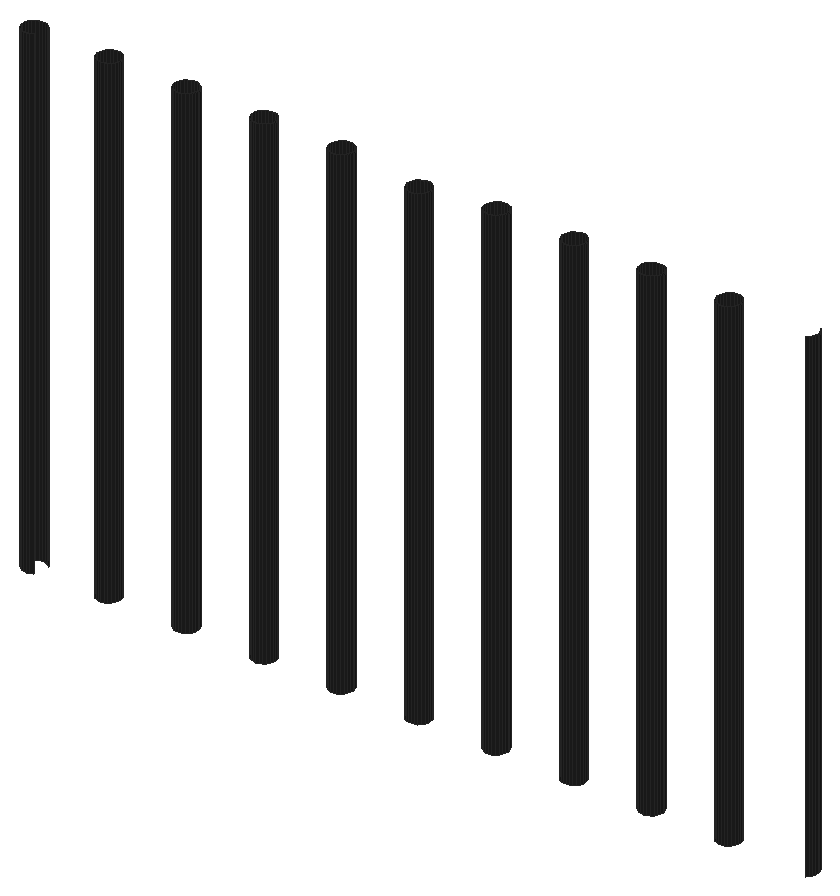
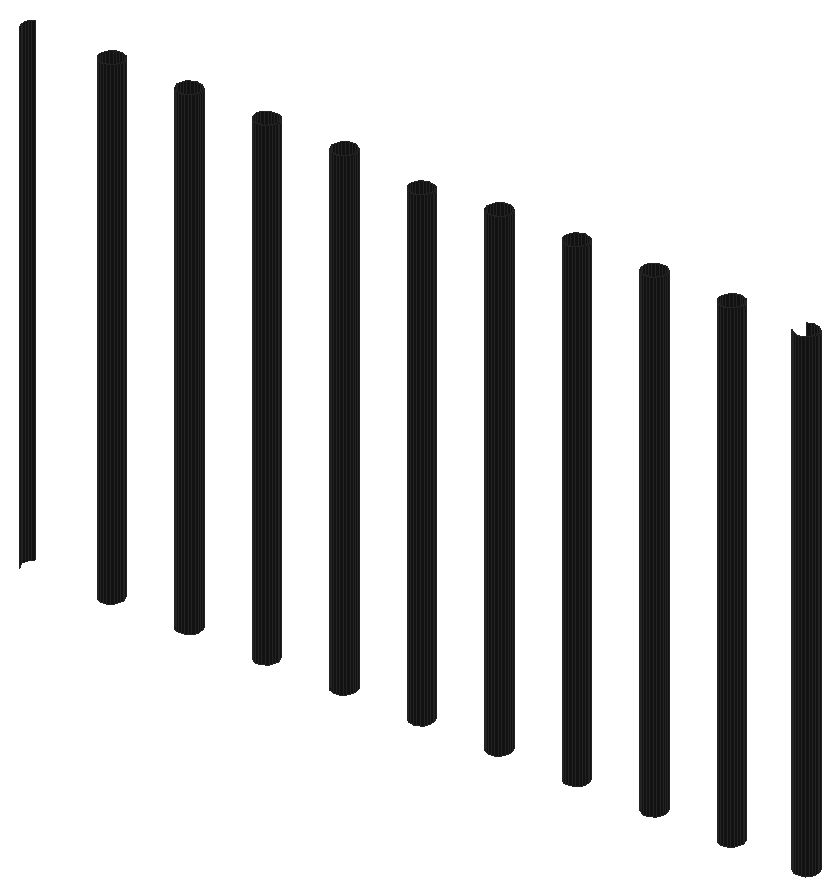
# SketchUp Ruby script. Lengths in inches.
U = 1.inch
M = Sketchup.active_model
def pt(a) = Geom::Point3d.new(a.map { |v| v * U })
def face(e, loops, mat)
  f = e.add_face(loops[0].map { |a| pt(a) })
  loops[1..].each { |l| e.add_face(l.map { |a| pt(a) }).erase! }
  f.material = f.back_material = mat if mat
  f
end
# faces: each face lists its corners as indices into pts; further lists are holes
def faces(e, pts, list, mat = nil) = list.each { |f| face(e, (f[0].is_a?(Array) ? f : [f]).map { |l| l.map { |i| pts[i] } }, mat) }
# xy, xz, yz: faces in a plane at the given z, y or x. An outline is a flat list of corners, or four numbers for a rectangle; further outlines are holes
def ring(l) = l.size == 4 ? [[l[0], l[1]], [l[2], l[1]], [l[2], l[3]], [l[0], l[3]]] : l.each_slice(2).to_a
def flat(e, list, mat, &to3) = list.each { |f| face(e, (f[0].is_a?(Array) ? f : [f]).map { |l| ring(l).map { |u, v| to3.(u, v) } }, mat) }
def xy(e, z, list, mat = nil) = flat(e, list, mat) { |x, y| [x, y, z] }
def xz(e, y, list, mat = nil) = flat(e, list, mat) { |x, z| [x, y, z] }
def yz(e, x, list, mat = nil) = flat(e, list, mat) { |y, z| [x, y, z] }
def lines(e, pts, list) = list.each { |a, b| e.add_line(pt(pts[a]), pt(pts[b])) }
# prism: a flat outline (further loops are holes) pulled along v
def prism(e, loops, v, mat = nil)
  f = face(e, loops, mat); d = Geom::Vector3d.new(v.map { |x| x * U })
  f.pushpull(f.normal.samedirection?(d) ? d.length : -d.length)
end
def box(e, o, s, mat = nil) = prism(e, [[o, [o[0] + s[0], o[1], o[2]], [o[0] + s[0], o[1] + s[1], o[2]], [o[0], o[1] + s[1], o[2]]]], [0, 0, s[2]], mat)
def at(x, y, z, deg = 0) = Geom::Transformation.translation(pt([x, y, z])) * Geom::Transformation.rotation(ORIGIN, Z_AXIS, deg.degrees)
def axes(o, x, y, z) = Geom::Transformation.new([*x, 0, *y, 0, *z, 0, *pt(o).to_a, 1])
def part(name) = M.definitions.add(name)
# library, detail: a bought-in or finely detailed component or shape, given as its bounding box
def library(name, o, s) = part(name).tap { |d| box(d.entities, o, s) }
def detail(e, o, s) = box(e.add_group.entities, o, s)
def put(e, d, t, mat = nil) = e.add_instance(d, t).tap { |i| i.material = mat if mat }
def group(e, t, mat = nil) = e.add_group.tap { |g| g.transformation = t; g.material = mat if mat }.entities
root = M.entities
M.materials.add("[Color M08]").color = [30, 30, 30]
xz(root,194.51,[[121.8,321,122,353.72],[126.86,321,127.06,353.72],[132.11,321,132.31,353.72],[137.36,321,137.56,353.72],[142.61,321,142.81,353.72],
  [147.86,321,148.06,353.1875],[153.11,321,153.31,353.72],[158.36,321,158.56,353.72],[163.61,321,163.81,353.72],[168.86,321,169.06,353.72]],"[Color M08]")
yz(root,126.24,[[195.18,321,195.375,353.72]],"[Color M08]")
yz(root,131.49,[[195.18,321,195.375,353.72]],"[Color M08]")
yz(root,136.74,[[195.18,321,195.375,353.72]],"[Color M08]")
yz(root,141.99,[[195.18,321,195.375,353.72]],"[Color M08]")
yz(root,147.24,[[195.18,321,195.375,353.1875]],"[Color M08]")
yz(root,152.49,[[195.18,321,195.375,353.72]],"[Color M08]")
yz(root,157.74,[[195.18,321,195.375,353.72]],"[Color M08]")
yz(root,162.99,[[195.18,321,195.375,353.72]],"[Color M08]")
yz(root,168.24,[[195.18,321,195.375,353.72]],"[Color M08]")
p = [[121.61,194.57,321],[121.8,194.51,321],[121.8,194.51,353.72],[121.61,194.57,353.72],[122,194.51,321],[122.1875,194.55,321],
  [122.1875,194.55,353.72],[122,194.51,353.72],[126.68,194.57,321],[126.86,194.51,321],[126.86,194.51,353.72],[126.68,194.57,353.72],
  [127.06,194.51,321],[127.25,194.55,321],[127.25,194.55,353.72],[127.06,194.51,353.72],[131.93,194.57,321],[132.11,194.51,321],
  [132.11,194.51,353.72],[131.93,194.57,353.72],[132.31,194.51,321],[132.5,194.55,321],[132.5,194.55,353.72],[132.31,194.51,353.72],
  [137.18,194.57,321],[137.36,194.51,321],[137.36,194.51,353.72],[137.18,194.57,353.72],[137.56,194.51,321],[137.75,194.55,321],
  [137.75,194.55,353.72],[137.56,194.51,353.72],[142.43,194.57,321],[142.61,194.51,321],[142.61,194.51,353.72],[142.43,194.57,353.72],
  [142.81,194.51,321],[143,194.55,321],[143,194.55,353.72],[142.81,194.51,353.72],[147.68,194.57,321],[147.86,194.51,321],
  [147.86,194.51,353.1875],[147.68,194.57,353.1875],[148.06,194.51,321],[148.25,194.55,321],[148.25,194.55,353.1875],[148.06,194.51,353.1875],
  [152.93,194.57,321],[153.11,194.51,321],[153.11,194.51,353.72],[152.93,194.57,353.72],[153.31,194.51,321],[153.5,194.55,321],
  [153.5,194.55,353.72],[153.31,194.51,353.72],[158.18,194.57,321],[158.36,194.51,321],[158.36,194.51,353.72],[158.18,194.57,353.72],
  [158.56,194.51,321],[158.75,194.55,321],[158.75,194.55,353.72],[158.56,194.51,353.72],[163.43,194.57,321],[163.61,194.51,321],
  [163.61,194.51,353.72],[163.43,194.57,353.72],[163.81,194.51,321],[164,194.55,321],[164,194.55,353.72],[163.81,194.51,353.72],
  [168.68,194.57,321],[168.86,194.51,321],[168.86,194.51,353.72],[168.68,194.57,353.72],[169.06,194.51,321],[169.25,194.55,321],
  [169.25,194.55,353.72],[169.06,194.51,353.72],[121.45,194.67,321],[121.45,194.67,353.72],[122.36,194.64,321],[122.36,194.64,353.72],
  [126.51,194.67,321],[126.51,194.67,353.72],[127.42,194.64,321],[127.42,194.64,353.72],[127.5625,194.78,321],[127.5625,194.78,353.72],
  [131.76,194.67,321],[131.76,194.67,353.72],[132.67,194.64,321],[132.67,194.64,353.72],[132.8125,194.78,321],[132.8125,194.78,353.72],
  [137.01,194.67,321],[137.01,194.67,353.72],[137.92,194.64,321],[137.92,194.64,353.72],[138.0625,194.78,321],[138.0625,194.78,353.72],
  [142.26,194.67,321],[142.26,194.67,353.72],[143.17,194.64,321],[143.17,194.64,353.72],[143.3125,194.78,321],[143.3125,194.78,353.72],
  [147.51,194.67,321],[147.51,194.67,353.1875],[148.42,194.64,321],[148.42,194.64,353.1875],[148.5625,194.78,321],[148.5625,194.78,353.1875],
  [152.76,194.67,321],[152.76,194.67,353.72],[153.67,194.64,321],[153.67,194.64,353.72],[153.8125,194.78,321],[153.8125,194.78,353.72],
  [158.01,194.67,321],[158.01,194.67,353.72],[158.92,194.64,321],[158.92,194.64,353.72],[159.0625,194.78,321],[159.0625,194.78,353.72],
  [163.26,194.67,321],[163.26,194.67,353.72],[164.17,194.64,321],[164.17,194.64,353.72],[164.3125,194.78,321],[164.3125,194.78,353.72],
  [168.51,194.67,321],[168.51,194.67,353.72],[169.42,194.64,321],[169.42,194.64,353.72],[169.5625,194.78,321],[169.5625,194.78,353.72],
  [174.67,194.64,321],[174.8125,194.78,321],[174.8125,194.78,353.72],[174.67,194.64,353.72],[121.3125,194.81,321],[121.3125,194.81,353.72],
  [126.375,194.81,321],[126.375,194.81,353.72],[131.625,194.81,321],[131.625,194.81,353.72],[136.875,194.81,321],[136.875,194.81,353.72],
  [142.125,194.81,321],[142.125,194.81,353.72],[147.375,194.81,321],[147.375,194.81,353.1875],[152.625,194.81,321],[152.625,194.81,353.72],
  [157.875,194.81,321],[157.875,194.81,353.72],[163.125,194.81,321],[163.125,194.81,353.72],[168.375,194.81,321],[168.375,194.81,353.72],
  [121.22,194.99,321],[121.22,194.99,353.72],[126.28,194.99,321],[126.28,194.99,353.72],[127.67,194.95,321],[127.67,194.95,353.72],
  [131.53,194.99,321],[131.53,194.99,353.72],[132.92,194.95,321],[132.92,194.95,353.72],[136.78,194.99,321],[136.78,194.99,353.72],
  [138.17,194.95,321],[138.17,194.95,353.72],[142.03,194.99,321],[142.03,194.99,353.72],[143.42,194.95,321],[143.42,194.95,353.72],
  [147.28,194.99,321],[147.28,194.99,353.1875],[148.67,194.95,321],[148.67,194.95,353.1875],[152.53,194.99,321],[152.53,194.99,353.72],
  [153.92,194.95,321],[153.92,194.95,353.72],[157.78,194.99,321],[157.78,194.99,353.72],[159.17,194.95,321],[159.17,194.95,353.72],
  [163.03,194.99,321],[163.03,194.99,353.72],[164.42,194.95,321],[164.42,194.95,353.72],[168.28,194.99,321],[168.28,194.99,353.72],
  [169.67,194.95,321],[169.67,194.95,353.72],[174.92,194.95,321],[174.92,194.95,353.72],[127.72,195.13,321],[127.72,195.13,353.72],
  [132.97,195.13,321],[132.97,195.13,353.72],[138.22,195.13,321],[138.22,195.13,353.72],[143.47,195.13,321],[143.47,195.13,353.72],
  [148.72,195.13,321],[148.72,195.13,353.1875],[153.97,195.13,321],[153.97,195.13,353.72],[159.22,195.13,321],[159.22,195.13,353.72],
  [164.47,195.13,321],[164.47,195.13,353.72],[169.72,195.13,321],[169.72,195.13,353.72],[174.97,195.13,321],[174.97,195.13,353.72],
  [121.17,195.18,321],[121.17,195.18,353.72],[126.24,195.18,321],[126.24,195.18,353.72],[131.49,195.18,321],[131.49,195.18,353.72],
  [136.74,195.18,321],[136.74,195.18,353.72],[141.99,195.18,321],[141.99,195.18,353.72],[147.24,195.18,321],[147.24,195.18,353.1875],
  [152.49,195.18,321],[152.49,195.18,353.72],[157.74,195.18,321],[157.74,195.18,353.72],[162.99,195.18,321],[162.99,195.18,353.72],
  [168.24,195.18,321],[168.24,195.18,353.72],[127.73,195.33,321],[127.73,195.33,353.72],[132.98,195.33,321],[132.98,195.33,353.72],
  [138.23,195.33,321],[138.23,195.33,353.72],[143.48,195.33,321],[143.48,195.33,353.72],[148.73,195.33,321],[148.73,195.33,353.1875],
  [153.98,195.33,321],[153.98,195.33,353.72],[159.23,195.33,321],[159.23,195.33,353.72],[164.48,195.33,321],[164.48,195.33,353.72],
  [169.73,195.33,321],[169.73,195.33,353.72],[174.98,195.33,321],[174.98,195.33,353.72],[121.18,195.375,321],[121.18,195.375,353.72],
  [127.68,195.52,321],[127.68,195.52,353.72],[132.93,195.52,321],[132.93,195.52,353.72],[138.18,195.52,321],[138.18,195.52,353.72],
  [143.43,195.52,321],[143.43,195.52,353.72],[148.68,195.52,321],[148.68,195.52,353.1875],[153.93,195.52,321],[153.93,195.52,353.72],
  [159.18,195.52,321],[159.18,195.52,353.72],[164.43,195.52,321],[164.43,195.52,353.72],[169.68,195.52,321],[169.68,195.52,353.72],
  [174.93,195.52,321],[174.93,195.52,353.72],[121.24,195.5625,321],[121.24,195.5625,353.72],[126.3,195.5625,321],[126.24,195.375,321],
  [126.24,195.375,353.72],[126.3,195.5625,353.72],[131.55,195.5625,321],[131.49,195.375,321],[131.49,195.375,353.72],[131.55,195.5625,353.72],
  [136.8,195.5625,321],[136.74,195.375,321],[136.74,195.375,353.72],[136.8,195.5625,353.72],[142.05,195.5625,321],[141.99,195.375,321],
  [141.99,195.375,353.72],[142.05,195.5625,353.72],[147.3,195.5625,321],[147.24,195.375,321],[147.24,195.375,353.1875],[147.3,195.5625,353.1875],
  [152.55,195.5625,321],[152.49,195.375,321],[152.49,195.375,353.72],[152.55,195.5625,353.72],[157.8,195.5625,321],[157.74,195.375,321],
  [157.74,195.375,353.72],[157.8,195.5625,353.72],[163.05,195.5625,321],[162.99,195.375,321],[162.99,195.375,353.72],[163.05,195.5625,353.72],
  [168.3,195.5625,321],[168.24,195.375,321],[168.24,195.375,353.72],[168.3,195.5625,353.72],[127.59,195.69,321],[127.59,195.69,353.72],
  [132.84,195.69,321],[132.84,195.69,353.72],[138.09,195.69,321],[138.09,195.69,353.72],[143.34,195.69,321],[143.34,195.69,353.72],
  [148.59,195.69,321],[148.59,195.69,353.1875],[153.84,195.69,321],[153.84,195.69,353.72],[159.09,195.69,321],[159.09,195.69,353.72],
  [164.34,195.69,321],[164.34,195.69,353.72],[169.59,195.69,321],[169.59,195.69,353.72],[174.84,195.69,321],[174.84,195.69,353.72],
  [121.34,195.73,321],[121.34,195.73,353.72],[126.4,195.73,321],[126.4,195.73,353.72],[131.65,195.73,321],[131.65,195.73,353.72],
  [136.9,195.73,321],[136.9,195.73,353.72],[142.15,195.73,321],[142.15,195.73,353.72],[147.4,195.73,321],[147.4,195.73,353.1875],
  [152.65,195.73,321],[152.65,195.73,353.72],[157.9,195.73,321],[157.9,195.73,353.72],[163.15,195.73,321],[163.15,195.73,353.72],
  [168.4,195.73,321],[168.4,195.73,353.72],[121.48,195.86,321],[121.48,195.86,353.72],[122.53,195.69,321],[122.4,195.83,321],
  [122.4,195.83,353.72],[122.53,195.69,353.72],[126.54,195.86,321],[126.54,195.86,353.72],[127.46,195.83,321],[127.46,195.83,353.72],
  [131.79,195.86,321],[131.79,195.86,353.72],[132.71,195.83,321],[132.71,195.83,353.72],[137.04,195.86,321],[137.04,195.86,353.72],
  [137.96,195.83,321],[137.96,195.83,353.72],[142.29,195.86,321],[142.29,195.86,353.72],[143.21,195.83,321],[143.21,195.83,353.72],
  [147.54,195.86,321],[147.54,195.86,353.1875],[148.46,195.83,321],[148.46,195.83,353.1875],[152.79,195.86,321],[152.79,195.86,353.72],
  [153.71,195.83,321],[153.71,195.83,353.72],[158.04,195.86,321],[158.04,195.86,353.72],[158.96,195.83,321],[158.96,195.83,353.72],
  [163.29,195.86,321],[163.29,195.86,353.72],[164.21,195.83,321],[164.21,195.83,353.72],[168.54,195.86,321],[168.54,195.86,353.72],
  [169.46,195.83,321],[169.46,195.83,353.72],[174.71,195.83,321],[174.71,195.83,353.72],[122.23,195.9375,321],[122.23,195.9375,353.72],
  [127.29,195.9375,321],[127.29,195.9375,353.72],[132.54,195.9375,321],[132.54,195.9375,353.72],[137.79,195.9375,321],[137.79,195.9375,353.72],
  [143.04,195.9375,321],[143.04,195.9375,353.72],[148.29,195.9375,321],[148.29,195.9375,353.1875],[153.54,195.9375,321],[153.54,195.9375,353.72],
  [158.79,195.9375,321],[158.79,195.9375,353.72],[164.04,195.9375,321],[164.04,195.9375,353.72],[169.29,195.9375,321],[169.29,195.9375,353.72],
  [121.65,195.95,321],[121.65,195.95,353.72],[122.04,195.99,321],[122.04,195.99,353.72],[126.72,195.95,321],[126.72,195.95,353.72],
  [127.1,195.99,321],[127.1,195.99,353.72],[131.97,195.95,321],[131.97,195.95,353.72],[132.35,195.99,321],[132.35,195.99,353.72],
  [137.22,195.95,321],[137.22,195.95,353.72],[137.6,195.99,321],[137.6,195.99,353.72],[142.47,195.95,321],[142.47,195.95,353.72],
  [142.85,195.99,321],[142.85,195.99,353.72],[147.72,195.95,321],[147.72,195.95,353.1875],[148.1,195.99,321],[148.1,195.99,353.1875],
  [152.97,195.95,321],[152.97,195.95,353.72],[153.35,195.99,321],[153.35,195.99,353.72],[158.22,195.95,321],[158.22,195.95,353.72],
  [158.6,195.99,321],[158.6,195.99,353.72],[163.47,195.95,321],[163.47,195.95,353.72],[163.85,195.99,321],[163.85,195.99,353.72],
  [168.72,195.95,321],[168.72,195.95,353.72],[169.1,195.99,321],[169.1,195.99,353.72],[121.85,196,321],[121.85,196,353.72],
  [126.91,196,321],[126.91,196,353.72],[132.16,196,321],[132.16,196,353.72],[137.41,196,321],[137.41,196,353.72],
  [142.66,196,321],[142.66,196,353.72],[147.91,196,321],[147.91,196,353.1875],[153.16,196,321],[153.16,196,353.72],
  [158.41,196,321],[158.41,196,353.72],[163.66,196,321],[163.66,196,353.72],[168.91,196,321],[168.91,196,353.72]]
faces(root,p,[[0,1,2,3],[4,5,6,7],[8,9,10,11],[12,13,14,15],[16,17,18,19],[20,21,22,23],[24,25,26,27],[28,29,30,31],
  [32,33,34,35],[36,37,38,39],[40,41,42,43],[44,45,46,47],[48,49,50,51],[52,53,54,55],[56,57,58,59],[60,61,62,63],
  [64,65,66,67],[68,69,70,71],[72,73,74,75],[76,77,78,79],[80,0,3,81],[5,82,83,6],[84,8,11,85],[13,86,87,14],
  [86,88,89,87],[90,16,19,91],[21,92,93,22],[92,94,95,93],[96,24,27,97],[29,98,99,30],[98,100,101,99],[102,32,35,103],
  [37,104,105,38],[104,106,107,105],[108,40,43,109],[45,110,111,46],[110,112,113,111],[114,48,51,115],[53,116,117,54],[116,118,119,117],
  [120,56,59,121],[61,122,123,62],[122,124,125,123],[126,64,67,127],[69,128,129,70],[128,130,131,129],[132,72,75,133],[77,134,135,78],
  [134,136,137,135],[138,139,140,141],[142,80,81,143],[144,84,85,145],[146,90,91,147],[148,96,97,149],[150,102,103,151],[152,108,109,153],
  [154,114,115,155],[156,120,121,157],[158,126,127,159],[160,132,133,161],[162,142,143,163],[164,144,145,165],[88,166,167,89],[168,146,147,169],
  [94,170,171,95],[172,148,149,173],[100,174,175,101],[176,150,151,177],[106,178,179,107],[180,152,153,181],[112,182,183,113],[184,154,155,185],
  [118,186,187,119],[188,156,157,189],[124,190,191,125],[192,158,159,193],[130,194,195,131],[196,160,161,197],[136,198,199,137],[139,200,201,140],
  [166,202,203,167],[170,204,205,171],[174,206,207,175],[178,208,209,179],[182,210,211,183],[186,212,213,187],[190,214,215,191],[194,216,217,195],
  [198,218,219,199],[200,220,221,201],[222,162,163,223],[224,164,165,225],[226,168,169,227],[228,172,173,229],[230,176,177,231],[232,180,181,233],
  [234,184,185,235],[236,188,189,237],[238,192,193,239],[240,196,197,241],[202,242,243,203],[204,244,245,205],[206,246,247,207],[208,248,249,209],
  [210,250,251,211],[212,252,253,213],[214,254,255,215],[216,256,257,217],[218,258,259,219],[220,260,261,221],[262,222,223,263],[242,264,265,243],
  [244,266,267,245],[246,268,269,247],[248,270,271,249],[250,272,273,251],[252,274,275,253],[254,276,277,255],[256,278,279,257],[258,280,281,259],
  [260,282,283,261],[284,262,263,285],[286,287,288,289],[290,291,292,293],[294,295,296,297],[298,299,300,301],[302,303,304,305],[306,307,308,309],
  [310,311,312,313],[314,315,316,317],[318,319,320,321],[264,322,323,265],[266,324,325,267],[268,326,327,269],[270,328,329,271],[272,330,331,273],
  [274,332,333,275],[276,334,335,277],[278,336,337,279],[280,338,339,281],[282,340,341,283],[342,284,285,343],[344,286,289,345],[346,290,293,347],
  [348,294,297,349],[350,298,301,351],[352,302,305,353],[354,306,309,355],[356,310,313,357],[358,314,317,359],[360,318,321,361],[362,342,343,363],
  [364,365,366,367],[368,344,345,369],[322,370,371,323],[372,346,347,373],[324,374,375,325],[376,348,349,377],[326,378,379,327],[380,350,351,381],
  [328,382,383,329],[384,352,353,385],[330,386,387,331],[388,354,355,389],[332,390,391,333],[392,356,357,393],[334,394,395,335],[396,358,359,397],
  [336,398,399,337],[400,360,361,401],[338,402,403,339],[340,404,405,341],[365,406,407,366],[370,408,409,371],[374,410,411,375],[378,412,413,379],
  [382,414,415,383],[386,416,417,387],[390,418,419,391],[394,420,421,395],[398,422,423,399],[402,424,425,403],[426,362,363,427],[406,428,429,407],
  [430,368,369,431],[408,432,433,409],[434,372,373,435],[410,436,437,411],[438,376,377,439],[412,440,441,413],[442,380,381,443],[414,444,445,415],
  [446,384,385,447],[416,448,449,417],[450,388,389,451],[418,452,453,419],[454,392,393,455],[420,456,457,421],[458,396,397,459],[422,460,461,423],
  [462,400,401,463],[424,464,465,425],[466,426,427,467],[428,466,467,429],[468,430,431,469],[432,468,469,433],[470,434,435,471],[436,470,471,437],
  [472,438,439,473],[440,472,473,441],[474,442,443,475],[444,474,475,445],[476,446,447,477],[448,476,477,449],[478,450,451,479],[452,478,479,453],
  [480,454,455,481],[456,480,481,457],[482,458,459,483],[460,482,483,461],[484,462,463,485],[464,484,485,465]],"[Color M08]")
